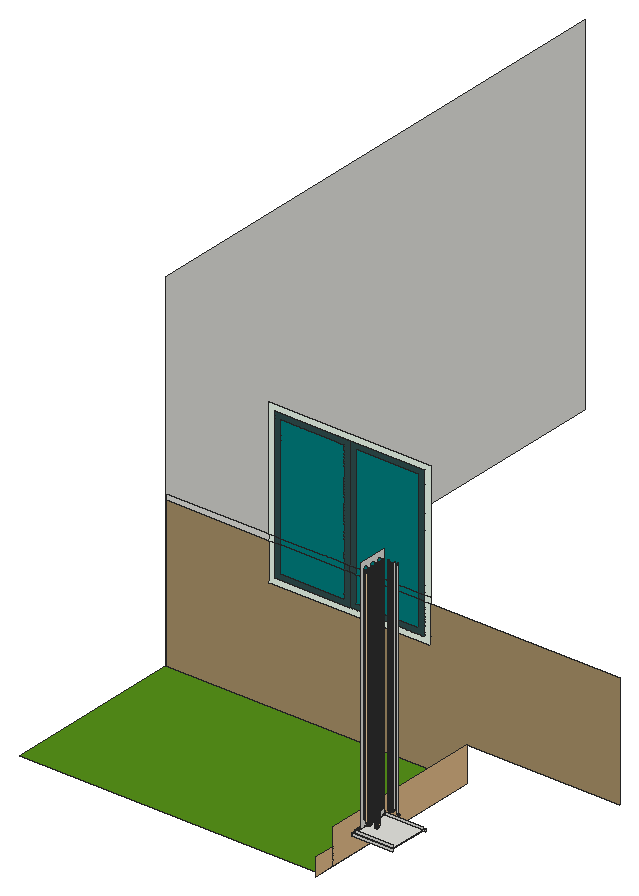
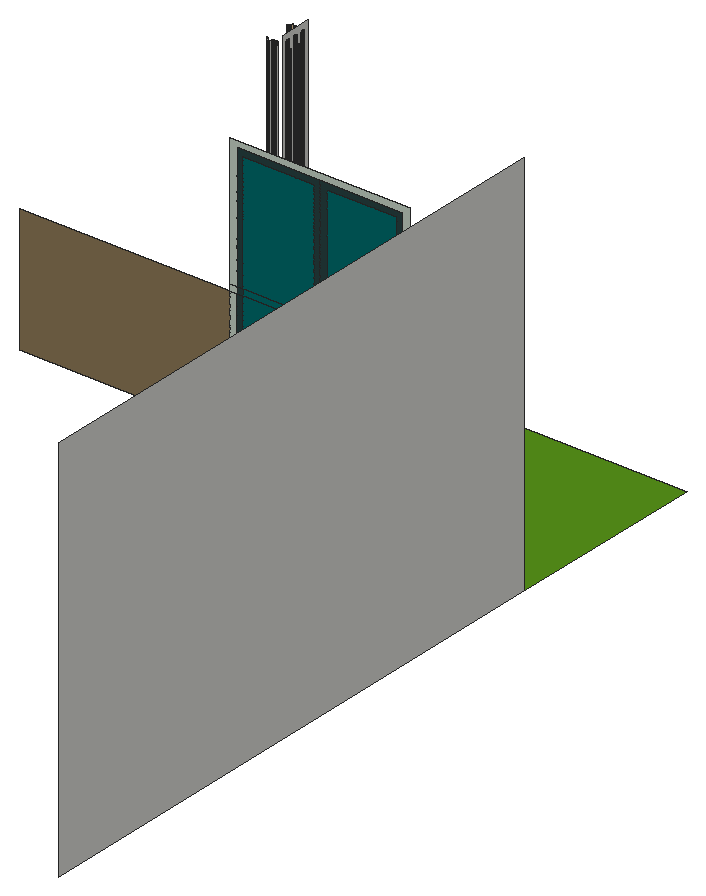
# SketchUp Ruby script. Lengths in inches.
U = 1.inch
M = Sketchup.active_model
def pt(a) = Geom::Point3d.new(a.map { |v| v * U })
def face(e, loops, mat)
  f = e.add_face(loops[0].map { |a| pt(a) })
  loops[1..].each { |l| e.add_face(l.map { |a| pt(a) }).erase! }
  f.material = f.back_material = mat if mat
  f
end
# faces: each face lists its corners as indices into pts; further lists are holes
def faces(e, pts, list, mat = nil) = list.each { |f| face(e, (f[0].is_a?(Array) ? f : [f]).map { |l| l.map { |i| pts[i] } }, mat) }
# xy, xz, yz: faces in a plane at the given z, y or x. An outline is a flat list of corners, or four numbers for a rectangle; further outlines are holes
def ring(l) = l.size == 4 ? [[l[0], l[1]], [l[2], l[1]], [l[2], l[3]], [l[0], l[3]]] : l.each_slice(2).to_a
def flat(e, list, mat, &to3) = list.each { |f| face(e, (f[0].is_a?(Array) ? f : [f]).map { |l| ring(l).map { |u, v| to3.(u, v) } }, mat) }
def xy(e, z, list, mat = nil) = flat(e, list, mat) { |x, y| [x, y, z] }
def xz(e, y, list, mat = nil) = flat(e, list, mat) { |x, z| [x, y, z] }
def yz(e, x, list, mat = nil) = flat(e, list, mat) { |y, z| [x, y, z] }
def lines(e, pts, list) = list.each { |a, b| e.add_line(pt(pts[a]), pt(pts[b])) }
# prism: a flat outline (further loops are holes) pulled along v
def prism(e, loops, v, mat = nil)
  f = face(e, loops, mat); d = Geom::Vector3d.new(v.map { |x| x * U })
  f.pushpull(f.normal.samedirection?(d) ? d.length : -d.length)
end
def box(e, o, s, mat = nil) = prism(e, [[o, [o[0] + s[0], o[1], o[2]], [o[0] + s[0], o[1] + s[1], o[2]], [o[0], o[1] + s[1], o[2]]]], [0, 0, s[2]], mat)
def at(x, y, z, deg = 0) = Geom::Transformation.translation(pt([x, y, z])) * Geom::Transformation.rotation(ORIGIN, Z_AXIS, deg.degrees)
def axes(o, x, y, z) = Geom::Transformation.new([*x, 0, *y, 0, *z, 0, *pt(o).to_a, 1])
def part(name) = M.definitions.add(name)
# library, detail: a bought-in or finely detailed component or shape, given as its bounding box
def library(name, o, s) = part(name).tap { |d| box(d.entities, o, s) }
def detail(e, o, s) = box(e.add_group.entities, o, s)
def put(e, d, t, mat = nil) = e.add_instance(d, t).tap { |i| i.material = mat if mat }
def group(e, t, mat = nil) = e.add_group.tap { |g| g.transformation = t; g.material = mat if mat }.entities
root = M.entities
M.materials.add("[0033_NavajoWhite]").color = [255, 222, 173]
M.materials.add("[0036_BurlyWood]").color = [222, 184, 135]
M.materials.add("[0066_Honeydew]").color = [240, 255, 240]
M.materials.add("[0078_DarkSlateGray]").color = [47, 79, 79]
M.materials.add("[0079_Teal]").color = [0, 128, 128]
M.materials.add("[Stone Sandstone Ashlar Light]").color = [168, 145, 104]
M.materials.add("[Vegetation Honey Locust]").color = [86, 145, 25]
xy(root,0,[[0,1.91,103.43,64.75]],"[Vegetation Honey Locust]")
xy(root,12.13,[[[109.69,7.58,123.72,21.61],[109.86,7.74,123.55,21.44]],[110.21,8.1,123.2,21.09]])
xz(root,7.58,[[109.69,11.46,123.72,12.13]])
xz(root,8.1,[[110.21,12.13,123.2,13.02]])
xz(root,21.09,[[110.21,12.13,123.2,13.02]])
xz(root,21.61,[[109.69,11.46,123.72,12.13]])
xz(root,64.75,[[0,51.19,35.4,53.19]])
xz(root,64.75,[[35.4,38.25,90.9,38.25,90.9,51.19,88.9,51.19,88.9,40.25,37.4,40.25,37.4,51.19,35.4,51.19],[35.4,51.19,37.4,53.19],[88.9,51.19,90.9,53.19],[35.4,53.19,37.4,53.19,37.4,91.75,88.9,91.75,88.9,53.19,90.9,53.19,90.9,93.75,35.4,93.75]],"[0066_Honeydew]")
xz(root,64.75,[[37.4,40.25,63.15,40.25,63.15,51.19,61.15,51.19,61.15,42.25,39.4,42.25,39.4,51.19,37.4,51.19],[63.15,40.25,88.9,40.25,88.9,51.19,86.9,51.19,86.9,42.25,65.15,42.25,65.15,51.19,63.15,51.19],[37.4,51.19,39.4,53.19],[61.15,51.19,63.15,53.19],[63.15,51.19,65.15,53.19],
  [86.9,51.19,88.9,53.19],[37.4,53.19,39.4,53.19,39.4,89.75,61.15,89.75,61.15,53.19,63.15,53.19,63.15,91.75,37.4,91.75],[63.15,53.19,65.15,53.19,65.15,89.75,86.9,89.75,86.9,53.19,88.9,53.19,88.9,91.75,63.15,91.75]],"[0078_DarkSlateGray]")
xz(root,64.75,[[39.4,42.25,61.15,51.19],[65.15,42.25,86.9,51.19],[39.4,51.19,61.15,53.19],[65.15,51.19,86.9,53.19],[39.4,53.19,61.15,89.75],
  [65.15,53.19,86.9,89.75]],"[0079_Teal]")
xz(root,64.75,[[0,0,103.43,0,103.43,12,155.99,12,155.99,51.19,90.9,51.19,90.9,38.25,35.4,38.25,35.4,51.19,0,51.19]],"[Stone Sandstone Ashlar Light]")
yz(root,0,[[64.75,0,244.75,120]])
yz(root,103.43,[[0,0,7.125,6],[7.125,0,64.75,12]],"[0036_BurlyWood]")
yz(root,109.69,[[7.58,11.46,21.61,12.13]])
yz(root,110.21,[[8.1,12.13,21.09,13.02],[8.1,13.02,21.09,13.17]])
yz(root,111,[[[9.67,13.17,19.51,94.95],[17.55,15.23,17.8,15.27,18.04,15.36,18.24,15.5,18.4,15.69,18.5,15.9,18.53,16.14,18.53,92.51,18.5,92.74,18.4,92.96,18.24,93.15,18.04,93.29,17.8,93.38,17.55,93.41,17.29,93.38,17.05,93.29,16.85,93.15,16.69,92.96,16.59,92.74,16.5625,92.51,16.5625,16.14,16.59,15.9,16.69,15.69,16.85,15.5,17.05,15.36,17.29,15.27],[14.59,15.23,14.85,15.27,15.08,15.36,15.29,15.5,15.44,15.69,15.54,15.9,15.58,16.14,15.58,92.51,15.54,92.74,15.44,92.96,15.29,93.15,15.08,93.29,14.85,93.38,14.59,93.41,14.34,93.38,14.1,93.29,13.9,93.15,13.74,92.96,13.64,92.74,13.61,92.51,13.61,16.14,13.64,15.9,13.74,15.69,13.9,15.5,14.1,15.36,14.34,15.27],[11.64,15.23,11.89,15.27,12.13,15.36,12.34,15.5,12.49,15.69,12.59,15.9,12.625,16.14,12.625,92.51,12.59,92.74,12.49,92.96,12.34,93.15,12.13,93.29,11.89,93.38,11.64,93.41,11.39,93.38,11.15,93.29,10.94,93.15,10.79,92.96,10.6875,92.74,10.66,92.51,10.66,16.14,10.6875,15.9,10.79,15.69,10.94,15.5,11.15,15.36,11.39,15.27]]])
p = [[109.89,7.78,12.15],[109.89,21.41,12.15],[109.86,21.44,12.13],[109.86,7.74,12.13],[123.55,7.74,12.13],[123.52,7.78,12.15],
  [109.95,7.84,12.2],[109.95,21.35,12.2],[110.01,7.9,12.27],[110.01,21.29,12.27],[110.0625,7.95,12.36],[110.0625,21.24,12.36],
  [110.11,8,12.47],[110.11,21.1875,12.47],[110.15,8.03,12.59],[110.15,21.15,12.59],[110.18,8.06,12.73],[110.18,21.12,12.73],
  [110.2,8.09,12.87],[110.2,21.1,12.87],[110.21,8.1,13.02],[110.21,21.09,13.02],[113.28,9.8,15.09],[113.26,9.67,15.09],
  [113.5,9.67,15],[113.51,9.74,15],[113.53,9.8,15],[113.33,9.92,15.09],[113.75,9.67,14.97],[113.57,9.85,15],
  [113.625,9.89,15],[113.6875,9.92,15],[113.75,9.93,15],[113.82,9.92,15],[113.88,9.89,15],[113.93,9.85,15],
  [113.97,9.8,15],[114,9.74,15],[114.01,9.67,15],[114.23,9.8,15.09],[114.18,9.92,15.09],[114.25,9.67,15.09],
  [116.23,9.8,15.09],[116.21,9.67,15.09],[116.45,9.67,15],[116.46,9.74,15],[116.49,9.8,15],[116.28,9.92,15.09],
  [116.71,9.67,14.97],[116.53,9.85,15],[116.58,9.89,15],[116.64,9.92,15],[116.71,9.93,15],[113.41,10.02,15.09],
  [114.1,10.02,15.09],[116.36,10.02,15.09],[113.51,10.1,15.09],[113.625,10.15,15.09],[113.75,10.16,15.09],[113.88,10.15,15.09],
  [114,10.1,15.09],[116.46,10.1,15.09],[116.58,10.15,15.09],[116.71,10.16,15.09],[113.625,19.29,15],[113.51,19.09,15.09],
  [113.625,19.04,15.09],[113.6875,19.27,15],[113.75,19.02,15.09],[113.75,19.26,15],[113.88,19.04,15.09],[113.82,19.27,15],
  [114,19.09,15.09],[113.88,19.29,15],[116.58,19.29,15],[116.46,19.09,15.09],[116.58,19.04,15.09],[116.64,19.27,15],
  [116.71,19.02,15.09],[116.71,19.26,15],[113.57,19.33,15],[113.41,19.17,15.09],[114.1,19.17,15.09],[113.93,19.33,15],
  [116.53,19.33,15],[116.36,19.17,15.09],[113.53,19.39,15],[113.33,19.27,15.09],[114.18,19.27,15.09],[113.97,19.39,15],
  [116.49,19.39,15],[116.28,19.27,15.09],[113.51,19.45,15],[113.28,19.39,15.09],[113.75,19.51,14.97],[114.23,19.39,15.09],
  [114,19.45,15],[116.46,19.45,15],[116.23,19.39,15.09],[116.71,19.51,14.97],[113.5,19.51,15],[113.26,19.51,15.09],
  [114.01,19.51,15],[114.25,19.51,15.09],[116.45,19.51,15],[116.21,19.51,15.09],[113.08,9.85,15.24],[113.06,9.67,15.24],
  [114.45,9.67,15.24],[114.43,9.85,15.24],[116.03,9.85,15.24],[116.01,9.67,15.24],[113.15,10.02,15.24],[114.36,10.02,15.24],
  [116.1,10.02,15.24],[113.26,10.16,15.24],[114.25,10.16,15.24],[116.21,10.16,15.24],[113.41,10.27,15.24],[114.1,10.27,15.24],
  [116.36,10.27,15.24],[113.57,10.34,15.24],[113.75,10.37,15.24],[113.93,10.34,15.24],[116.53,10.34,15.24],[116.71,10.37,15.24],
  [113.41,18.91,15.24],[113.57,18.84,15.24],[113.75,18.82,15.24],[113.93,18.84,15.24],[114.1,18.91,15.24],[116.36,18.91,15.24],
  [116.53,18.84,15.24],[116.71,18.82,15.24],[113.26,19.02,15.24],[114.25,19.02,15.24],[116.21,19.02,15.24],[113.15,19.17,15.24],
  [114.36,19.17,15.24],[116.1,19.17,15.24],[113.08,19.33,15.24],[114.43,19.33,15.24],[116.03,19.33,15.24],[113.06,19.51,15.24],
  [114.45,19.51,15.24],[116.01,19.51,15.24],[112.93,9.89,15.42],[112.9,9.67,15.42],[114.61,9.67,15.42],[114.58,9.89,15.42],
  [115.88,9.89,15.42],[115.85,9.67,15.42],[113.01,10.1,15.42],[114.49,10.1,15.42],[115.97,10.1,15.42],[113.15,10.27,15.42],
  [114.36,10.27,15.42],[116.1,10.27,15.42],[113.33,10.41,15.42],[114.18,10.41,15.42],[116.28,10.41,15.42],[113.53,10.49,15.42],
  [113.75,10.52,15.42],[113.97,10.49,15.42],[116.49,10.49,15.42],[116.71,10.52,15.42],[111.0625,11.39,15.27],[111,11.64,15.23],
  [111,11.39,15.27],[111.125,11.42,15.27],[111.18,11.46,15.27],[111.22,11.51,15.27],[111.24,11.57,15.27],[111.0625,11.89,15.27],
  [111,11.89,15.27],[111.125,11.86,15.27],[111.18,11.82,15.27],[111.22,11.77,15.27],[111.24,11.71,15.27],[111.25,11.64,15.27],
  [111.0625,14.35,15.27],[111,14.59,15.23],[111,14.34,15.27],[111.125,14.37,15.27],[111.18,14.41,15.27],[111.22,14.47,15.27],
  [111.24,14.53,15.27],[111.25,14.59,15.27],[111.0625,14.84,15.27],[111,14.85,15.27],[111.125,14.8125,15.27],[111.18,14.77,15.27],
  [111.22,14.72,15.27],[111.24,14.66,15.27],[111,17.29,15.27],[111.0625,17.3,15.27],[111,17.55,15.23],[111.125,17.32,15.27],
  [111.18,17.37,15.27],[111.22,17.42,15.27],[111.24,17.48,15.27],[111.0625,17.79,15.27],[111,17.8,15.27],[111.125,17.77,15.27],
  [111.18,17.73,15.27],[111.22,17.67,15.27],[111.24,17.61,15.27],[111.25,17.55,15.27],[113.33,18.78,15.42],[113.53,18.69,15.42],
  [113.75,18.66,15.42],[113.97,18.69,15.42],[114.18,18.78,15.42],[116.28,18.78,15.42],[116.49,18.69,15.42],[116.71,18.66,15.42],
  [113.15,18.91,15.42],[114.36,18.91,15.42],[116.1,18.91,15.42],[113.01,19.09,15.42],[114.49,19.09,15.42],[115.97,19.09,15.42],
  [112.93,19.29,15.42],[114.58,19.29,15.42],[115.88,19.29,15.42],[112.9,19.51,15.42],[114.61,19.51,15.42],[115.85,19.51,15.42],
  [111,11.15,15.36],[111.125,11.16,15.36],[111.24,11.21,15.36],[111.35,11.29,15.36],[111.42,11.39,15.36],[111.47,11.51,15.36],
  [111.49,11.64,15.36],[111.47,11.77,15.36],[111.42,11.89,15.36],[111.35,11.99,15.36],[111.24,12.07,15.36],[111.125,12.12,15.36],
  [111,12.13,15.36],[111,14.1,15.36],[111.125,14.12,15.36],[111.24,14.17,15.36],[111.35,14.24,15.36],[111.42,14.35,15.36],
  [111.47,14.47,15.36],[111.49,14.59,15.36],[111.47,14.72,15.36],[111.42,14.84,15.36],[111.35,14.94,15.36],[111.125,15.07,15.36],
  [111,15.08,15.36],[111.24,15.02,15.36],[111,17.05,15.36],[111.125,17.07,15.36],[111.24,17.12,15.36],[111.35,17.2,15.36],
  [111.42,17.3,15.36],[111.47,17.42,15.36],[111.49,17.55,15.36],[111.47,17.67,15.36],[111.42,17.79,15.36],[111.24,17.97,15.36],
  [111.35,17.89,15.36],[111.125,18.02,15.36],[111,18.04,15.36],[112.83,9.92,15.64],[112.8,9.67,15.64],[114.7,9.67,15.64],
  [114.67,9.92,15.64],[115.79,9.92,15.64],[115.76,9.67,15.64],[112.93,10.15,15.64],[114.58,10.15,15.64],[115.88,10.15,15.64],
  [113.08,10.34,15.64],[114.43,10.34,15.64],[116.03,10.34,15.64],[113.28,10.49,15.64],[114.23,10.49,15.64],[116.23,10.49,15.64],
  [113.51,10.59,15.64],[114,10.59,15.64],[116.46,10.59,15.64],[113.75,10.62,15.64],[116.71,10.62,15.64],[111,10.94,15.5],
  [111.18,10.97,15.5],[111.35,11.04,15.5],[111.49,11.15,15.5],[111.6,11.29,15.5],[111.67,11.46,15.5],[111.69,11.64,15.5],
  [111.67,11.82,15.5],[111.6,11.99,15.5],[111.49,12.13,15.5],[111.35,12.24,15.5],[111.18,12.3125,15.5],[111,12.34,15.5],
  [111,13.9,15.5],[111.18,13.92,15.5],[111.35,13.99,15.5],[111.49,14.1,15.5],[111.6,14.24,15.5],[111.67,14.41,15.5],
  [111.69,14.59,15.5],[111.67,14.77,15.5],[111.6,14.94,15.5],[111.49,15.08,15.5],[111.35,15.2,15.5],[111.18,15.26,15.5],
  [111,15.29,15.5],[111,16.85,15.5],[111.18,16.875,15.5],[111.35,16.94,15.5],[111.49,17.05,15.5],[111.6,17.2,15.5],
  [111.67,17.37,15.5],[111.69,17.55,15.5],[111.67,17.73,15.5],[111.6,17.89,15.5],[111.49,18.04,15.5],[111.35,18.15,15.5],
  [111.18,18.22,15.5],[111,18.24,15.5],[113.28,18.69,15.64],[113.51,18.6,15.64],[113.75,18.5625,15.64],[114,18.6,15.64],
  [114.23,18.69,15.64],[116.23,18.69,15.64],[116.46,18.6,15.64],[116.71,18.5625,15.64],[113.08,18.84,15.64],[114.43,18.84,15.64],
  [116.03,18.84,15.64],[112.93,19.04,15.64],[114.58,19.04,15.64],[115.88,19.04,15.64],[112.83,19.27,15.64],[114.67,19.27,15.64],
  [115.79,19.27,15.64],[112.8,19.51,15.64],[114.7,19.51,15.64],[115.76,19.51,15.64],[111,10.79,15.69],[111.22,10.82,15.69],
  [111.42,10.9,15.69],[111.6,11.04,15.69],[111.74,11.21,15.69],[111.82,11.42,15.69],[111.85,11.64,15.69],[111.82,11.86,15.69],
  [111.74,12.07,15.69],[111.6,12.24,15.69],[111.42,12.38,15.69],[111.22,12.46,15.69],[111,12.49,15.69],[111,13.74,15.69],
  [111.22,13.77,15.69],[111.42,13.85,15.69],[111.6,13.99,15.69],[111.74,14.17,15.69],[111.82,14.37,15.69],[111.85,14.59,15.69],
  [111.82,14.8125,15.69],[111.74,15.02,15.69],[111.6,15.2,15.69],[111.42,15.33,15.69],[111.22,15.42,15.69],[111,15.44,15.69],
  [111,16.69,15.69],[111.22,16.72,15.69],[111.42,16.81,15.69],[111.6,16.94,15.69],[111.74,17.12,15.69],[111.82,17.32,15.69],
  [111.85,17.55,15.69],[111.82,17.77,15.69],[111.74,17.97,15.69],[111.6,18.15,15.69],[111.42,18.28,15.69],[111.22,18.37,15.69],
  [111,18.4,15.69],[112.8,9.93,15.875],[112.77,9.67,15.875],[114.74,9.67,15.875],[114.7,9.93,15.875],[115.76,9.93,15.875],
  [115.72,9.67,15.875],[112.9,10.16,15.875],[114.61,10.16,15.875],[115.85,10.16,15.875],[113.06,10.37,15.875],[114.45,10.37,15.875],
  [116.01,10.37,15.875],[113.26,10.52,15.875],[114.25,10.52,15.875],[116.21,10.52,15.875],[113.5,10.62,15.875],[114.01,10.62,15.875],
  [116.45,10.62,15.875],[113.75,10.66,15.875],[116.71,10.66,15.875],[113.5,18.5625,15.875],[113.75,18.53,15.875],[114.01,18.5625,15.875],
  [116.45,18.5625,15.875],[116.71,18.53,15.875],[113.26,18.66,15.875],[114.25,18.66,15.875],[116.21,18.66,15.875],[113.06,18.82,15.875],
  [114.45,18.82,15.875],[116.01,18.82,15.875],[112.9,19.02,15.875],[114.61,19.02,15.875],[115.85,19.02,15.875],[112.8,19.26,15.875],
  [114.7,19.26,15.875],[115.76,19.26,15.875],[112.77,19.51,15.875],[114.74,19.51,15.875],[115.72,19.51,15.875],[111,10.6875,15.9],
  [111.24,10.72,15.9],[111.47,10.82,15.9],[111.67,10.97,15.9],[111.82,11.16,15.9],[111.92,11.39,15.9],[111.95,11.64,15.9],
  [111.92,11.89,15.9],[111.82,12.12,15.9],[111.67,12.3125,15.9],[111.47,12.46,15.9],[111.24,12.56,15.9],[111,12.59,15.9],
  [111,13.64,15.9],[111.24,13.67,15.9],[111.47,13.77,15.9],[111.67,13.92,15.9],[111.82,14.12,15.9],[111.92,14.35,15.9],
  [111.95,14.59,15.9],[111.92,14.84,15.9],[111.82,15.07,15.9],[111.67,15.26,15.9],[111.47,15.42,15.9],[111.24,15.51,15.9],
  [111,15.54,15.9],[111,16.59,15.9],[111.24,16.625,15.9],[111.47,16.72,15.9],[111.67,16.875,15.9],[111.82,17.07,15.9],
  [111.92,17.3,15.9],[111.95,17.55,15.9],[111.92,17.79,15.9],[111.82,18.02,15.9],[111.67,18.22,15.9],[111.47,18.37,15.9],
  [111.24,18.46,15.9],[111,18.5,15.9],[112.8,9.93,92.25],[112.77,9.67,92.25],[114.74,9.67,92.25],[114.7,9.93,92.25],
  [115.76,9.93,92.25],[115.72,9.67,92.25],[112.9,10.16,92.25],[114.61,10.16,92.25],[115.85,10.16,92.25],[113.06,10.37,92.25],
  [114.45,10.37,92.25],[116.01,10.37,92.25],[113.26,10.52,92.25],[114.25,10.52,92.25],[116.21,10.52,92.25],[113.5,10.62,92.25],
  [114.01,10.62,92.25],[116.45,10.62,92.25],[113.75,10.66,92.25],[116.71,10.66,92.25],[111,10.66,16.14],[111.25,10.6875,16.14],
  [111.49,10.79,16.14],[111.69,10.94,16.14],[111.85,11.15,16.14],[111.95,11.39,16.14],[111.98,11.64,16.14],[111.95,11.89,16.14],
  [111.85,12.13,16.14],[111.69,12.34,16.14],[111.49,12.49,16.14],[111.25,12.59,16.14],[111,12.625,16.14],[111,13.61,16.14],
  [111.25,13.64,16.14],[111.49,13.74,16.14],[111.69,13.9,16.14],[111.85,14.1,16.14],[111.95,14.34,16.14],[111.98,14.59,16.14],
  [111.95,14.85,16.14],[111.85,15.08,16.14],[111.69,15.29,16.14],[111.49,15.44,16.14],[111.25,15.54,16.14],[111,15.58,16.14],
  [111,16.5625,16.14],[111.25,16.59,16.14],[111.49,16.69,16.14],[111.69,16.85,16.14],[111.85,17.05,16.14],[111.95,17.29,16.14],
  [111.98,17.55,16.14],[111.95,17.8,16.14],[111.85,18.04,16.14],[111.69,18.24,16.14],[111.49,18.4,16.14],[111.25,18.5,16.14],
  [111,18.53,16.14],[113.5,18.5625,92.25],[113.75,18.53,92.25],[114.01,18.5625,92.25],[116.45,18.5625,92.25],[116.71,18.53,92.25],
  [113.26,18.66,92.25],[114.25,18.66,92.25],[116.21,18.66,92.25],[113.06,18.82,92.25],[114.45,18.82,92.25],[116.01,18.82,92.25],
  [112.9,19.02,92.25],[114.61,19.02,92.25],[115.85,19.02,92.25],[112.8,19.26,92.25],[114.7,19.26,92.25],[115.76,19.26,92.25],
  [112.77,19.51,92.25],[114.74,19.51,92.25],[115.72,19.51,92.25],[111,10.66,92.51],[111.25,10.6875,92.51],[111.49,10.79,92.51],
  [111.69,10.94,92.51],[111.85,11.15,92.51],[111.95,11.39,92.51],[111.98,11.64,92.51],[111.95,11.89,92.51],[111.85,12.13,92.51],
  [111.69,12.34,92.51],[111.49,12.49,92.51],[111.25,12.59,92.51],[111,12.625,92.51],[111,13.61,92.51],[111.25,13.64,92.51],
  [111.49,13.74,92.51],[111.69,13.9,92.51],[111.85,14.1,92.51],[111.95,14.34,92.51],[111.98,14.59,92.51],[111.95,14.85,92.51],
  [111.85,15.08,92.51],[111.69,15.29,92.51],[111.49,15.44,92.51],[111.25,15.54,92.51],[111,15.58,92.51],[111,16.5625,92.51],
  [111.25,16.59,92.51],[111.49,16.69,92.51],[111.69,16.85,92.51],[111.85,17.05,92.51],[111.95,17.29,92.51],[111.98,17.55,92.51],
  [111.95,17.8,92.51],[111.85,18.04,92.51],[111.69,18.24,92.51],[111.49,18.4,92.51],[111.25,18.5,92.51],[111,18.53,92.51]]
faces(root,p,[[0,1,2,3],[4,5,0,3],[6,7,1,0],[8,9,7,6],[10,11,9,8],[12,13,11,10],[14,15,13,12],[16,17,15,14],
  [18,19,17,16],[20,21,19,18],[64,65,66,67],[67,66,68,69],[69,68,70,71],[71,70,72,73],[74,75,76,77],[77,76,78,79],
  [80,81,65,64],[73,72,82,83],[84,85,75,74],[86,87,81,80],[83,82,88,89],[90,91,85,84],[92,93,87,86],[94,86,80],
  [94,80,64],[94,64,67],[94,67,69],[94,69,71],[94,71,73],[94,73,83],[94,83,89],[89,88,95,96],
  [97,98,91,90],[99,90,84],[99,84,74],[99,74,77],[99,77,79],[92,100,101,93],[92,94,100],[94,92,86],
  [94,89,96],[96,102,94],[95,103,102,96],[97,104,105,98],[97,99,104],[99,97,90],[65,126,127,66],[66,127,128,68],
  [68,128,129,70],[70,129,130,72],[75,131,132,76],[76,132,133,78],[81,134,126,65],[72,130,135,82],[85,136,131,75],[87,137,134,81],
  [82,135,138,88],[91,139,136,85],[93,140,137,87],[88,138,141,95],[98,142,139,91],[93,101,143,140],[141,144,103,95],[98,105,145,142],
  [166,167,168],[167,166,169],[167,169,170],[167,170,171],[167,171,172],[173,174,167],[167,175,173],[167,176,175],
  [167,177,176],[167,178,177],[167,179,178],[167,172,179],[180,181,182],[181,180,183],[181,183,184],[181,184,185],
  [181,185,186],[181,186,187],[188,189,181],[181,190,188],[181,191,190],[181,192,191],[181,193,192],[181,187,193],
  [194,195,196],[197,196,195],[198,196,197],[199,196,198],[200,196,199],[196,201,202],[201,196,203],[203,196,204],
  [204,196,205],[205,196,206],[207,196,200],[206,196,207],[126,208,209,127],[127,209,210,128],[128,210,211,129],[129,211,212,130],
  [131,213,214,132],[132,214,215,133],[134,216,208,126],[130,212,217,135],[136,218,213,131],[137,219,216,134],[135,217,220,138],[139,221,218,136],
  [140,222,219,137],[138,220,223,141],[142,224,221,139],[140,143,225,222],[223,226,144,141],[142,145,227,224],[166,168,228,229],[166,229,230,169],
  [169,230,231,170],[170,231,232,171],[171,232,233,172],[172,233,234,179],[179,234,235,178],[178,235,236,177],[176,237,238,175],[177,236,237,176],
  [239,240,174,173],[175,238,239,173],[180,182,241,242],[180,242,243,183],[183,243,244,184],[184,244,245,185],[185,245,246,186],[186,246,247,187],
  [187,247,248,193],[192,249,250,191],[193,248,249,192],[251,252,189,188],[190,253,251,188],[191,250,253,190],[254,255,195,194],[256,197,195,255],
  [257,198,197,256],[258,199,198,257],[259,200,199,258],[260,207,200,259],[261,206,207,260],[262,205,206,261],[263,203,204,264],[264,204,205,262],
  [202,201,265,266],[265,201,203,263],[229,228,287,288],[229,288,289,230],[230,289,290,231],[231,290,291,232],[232,291,292,233],[233,292,293,234],
  [234,293,294,235],[235,294,295,236],[236,295,296,237],[237,296,297,238],[298,299,240,239],[238,297,298,239],[242,241,300,301],[242,301,302,243],
  [243,302,303,244],[244,303,304,245],[245,304,305,246],[246,305,306,247],[247,306,307,248],[248,307,308,249],[249,308,309,250],[250,309,310,253],
  [253,310,311,251],[311,312,252,251],[313,314,255,254],[315,256,255,314],[316,257,256,315],[317,258,257,316],[318,259,258,317],[319,260,259,318],
  [320,261,260,319],[321,262,261,320],[322,264,262,321],[323,263,264,322],[266,265,324,325],[324,265,263,323],[208,326,327,209],[209,327,328,210],
  [210,328,329,211],[211,329,330,212],[213,331,332,214],[214,332,333,215],[216,334,326,208],[212,330,335,217],[218,336,331,213],[219,337,334,216],
  [217,335,338,220],[221,339,336,218],[222,340,337,219],[220,338,341,223],[224,342,339,221],[222,225,343,340],[341,344,226,223],[224,227,345,342],
  [288,287,346,347],[288,347,348,289],[289,348,349,290],[290,349,350,291],[291,350,351,292],[292,351,352,293],[293,352,353,294],[294,353,354,295],
  [295,354,355,296],[296,355,356,297],[297,356,357,298],[357,358,299,298],[301,300,359,360],[301,360,361,302],[302,361,362,303],[303,362,363,304],
  [304,363,364,305],[305,364,365,306],[306,365,366,307],[307,366,367,308],[308,367,368,309],[309,368,369,310],[310,369,370,311],[370,371,312,311],
  [372,373,314,313],[374,315,314,373],[375,316,315,374],[376,317,316,375],[377,318,317,376],[378,319,318,377],[379,320,319,378],[380,321,320,379],
  [381,322,321,380],[382,323,322,381],[383,324,323,382],[325,324,383,384],[327,405,406,328],[328,406,407,329],[332,408,409,333],[326,410,405,327],
  [329,407,411,330],[331,412,408,332],[334,413,410,326],[330,411,414,335],[336,415,412,331],[337,416,413,334],[335,414,417,338],[339,418,415,336],
  [340,419,416,337],[338,417,420,341],[342,421,418,339],[340,343,422,419],[420,423,344,341],[342,345,424,421],[347,346,425,426],[347,426,427,348],
  [348,427,428,349],[349,428,429,350],[350,429,430,351],[351,430,431,352],[352,431,432,353],[353,432,433,354],[354,433,434,355],[355,434,435,356],
  [356,435,436,357],[436,437,358,357],[360,359,438,439],[360,439,440,361],[361,440,441,362],[362,441,442,363],[363,442,443,364],[364,443,444,365],
  [365,444,445,366],[366,445,446,367],[367,446,447,368],[368,447,448,369],[369,448,449,370],[449,450,371,370],[451,452,373,372],[453,374,373,452],
  [454,375,374,453],[455,376,375,454],[456,377,376,455],[457,378,377,456],[458,379,378,457],[459,380,379,458],[460,381,380,459],[461,382,381,460],
  [462,383,382,461],[384,383,462,463],[426,425,484,485],[426,485,486,427],[427,486,487,428],[428,487,488,429],[429,488,489,430],[430,489,490,431],
  [431,490,491,432],[432,491,492,433],[433,492,493,434],[434,493,494,435],[435,494,495,436],[495,496,437,436],[439,438,497,498],[439,498,499,440],
  [440,499,500,441],[441,500,501,442],[442,501,502,443],[443,502,503,444],[444,503,504,445],[445,504,505,446],[446,505,506,447],[447,506,507,448],
  [448,507,508,449],[508,509,450,449],[510,511,452,451],[512,453,452,511],[513,454,453,512],[514,455,454,513],[515,456,455,514],[516,457,456,515],
  [517,458,457,516],[518,459,458,517],[519,460,459,518],[520,461,460,519],[521,462,461,520],[463,462,521,522],[406,405,523,524],[407,406,524,525],
  [409,408,526,527],[405,410,528,523],[411,407,525,529],[408,412,530,526],[410,413,531,528],[414,411,529,532],[412,415,533,530],[413,416,534,531],
  [417,414,532,535],[415,418,536,533],[416,419,537,534],[420,417,535,538],[418,421,539,536],[419,422,540,537],[423,420,538,541],[421,424,542,539],
  [485,484,543,544],[486,485,544,545],[487,486,545,546],[488,487,546,547],[489,488,547,548],[490,489,548,549],[491,490,549,550],[492,491,550,551],
  [493,492,551,552],[494,493,552,553],[495,494,553,554],[496,495,554,555],[498,497,556,557],[499,498,557,558],[500,499,558,559],[501,500,559,560],
  [502,501,560,561],[503,502,561,562],[504,503,562,563],[505,504,563,564],[506,505,564,565],[507,506,565,566],[508,507,566,567],[509,508,567,568],
  [511,510,569,570],[512,511,570,571],[513,512,571,572],[514,513,572,573],[515,514,573,574],[516,515,574,575],[517,516,575,576],[518,517,576,577],
  [519,518,577,578],[520,519,578,579],[521,520,579,580],[522,521,580,581]])
faces(root,p,[[22,23,24,25],[26,27,22,25],[25,24,28],[28,26,25],[28,29,26],[28,30,29],[28,31,30],[28,32,31],
  [28,33,32],[28,34,33],[28,35,34],[28,36,35],[28,37,36],[37,28,38],[37,39,40,36],[37,38,41,39],
  [42,43,44,45],[46,47,42,45],[45,44,48],[48,46,45],[48,49,46],[48,50,49],[48,51,50],[48,52,51],
  [29,53,27,26],[36,40,54,35],[49,55,47,46],[30,56,53,29],[31,57,56,30],[32,58,57,31],[33,59,58,32],[34,60,59,33],
  [35,54,60,34],[50,61,55,49],[51,62,61,50],[52,63,62,51],[106,107,23,22],[39,41,108,109],[110,111,43,42],[27,112,106,22],
  [39,109,113,40],[47,114,110,42],[53,115,112,27],[40,113,116,54],[55,117,114,47],[56,118,115,53],[54,116,119,60],[61,120,117,55],
  [57,121,118,56],[58,122,121,57],[59,123,122,58],[60,119,123,59],[62,124,120,61],[63,125,124,62],[146,147,107,106],[109,108,148,149],
  [150,151,111,110],[112,152,146,106],[109,149,153,113],[114,154,150,110],[115,155,152,112],[113,153,156,116],[117,157,154,114],[118,158,155,115],
  [116,156,159,119],[120,160,157,117],[121,161,158,118],[122,162,161,121],[123,163,162,122],[119,159,163,123],[124,164,160,120],[125,165,164,124],
  [267,268,147,146],[149,148,269,270],[271,272,151,150],[152,273,267,146],[149,270,274,153],[154,275,271,150],[155,276,273,152],[153,274,277,156],
  [157,278,275,154],[158,279,276,155],[156,277,280,159],[160,281,278,157],[161,282,279,158],[159,280,283,163],[164,284,281,160],[162,285,282,161],
  [163,283,285,162],[165,286,284,164],[385,386,268,267],[270,269,387,388],[389,390,272,271],[273,391,385,267],[270,388,392,274],[275,393,389,271],
  [276,394,391,273],[274,392,395,277],[278,396,393,275],[279,397,394,276],[277,395,398,280],[281,399,396,278],[282,400,397,279],[280,398,401,283],
  [284,402,399,281],[285,403,400,282],[283,401,403,285],[286,404,402,284],[386,385,464,465],[388,387,466,467],[390,389,468,469],[385,391,470,464],
  [392,388,467,471],[389,393,472,468],[391,394,473,470],[395,392,471,474],[393,396,475,472],[394,397,476,473],[398,395,474,477],[396,399,478,475],
  [397,400,479,476],[401,398,477,480],[399,402,481,478],[400,403,482,479],[403,401,480,482],[402,404,483,481]],"[0033_NavajoWhite]")
